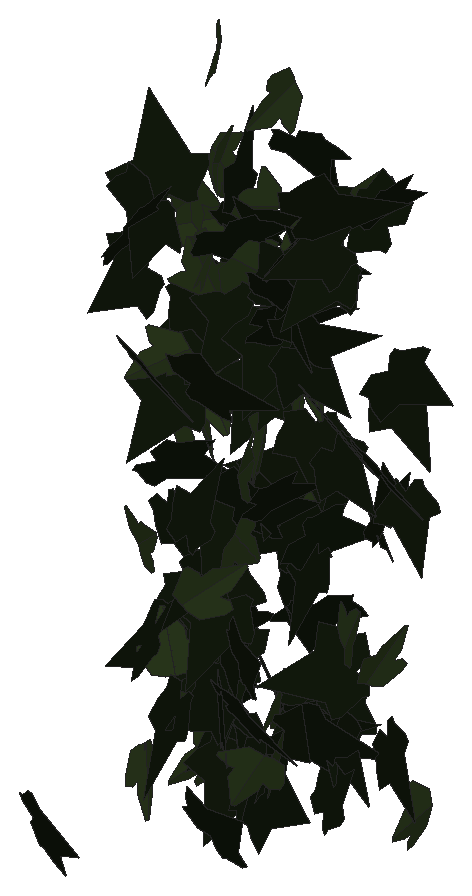
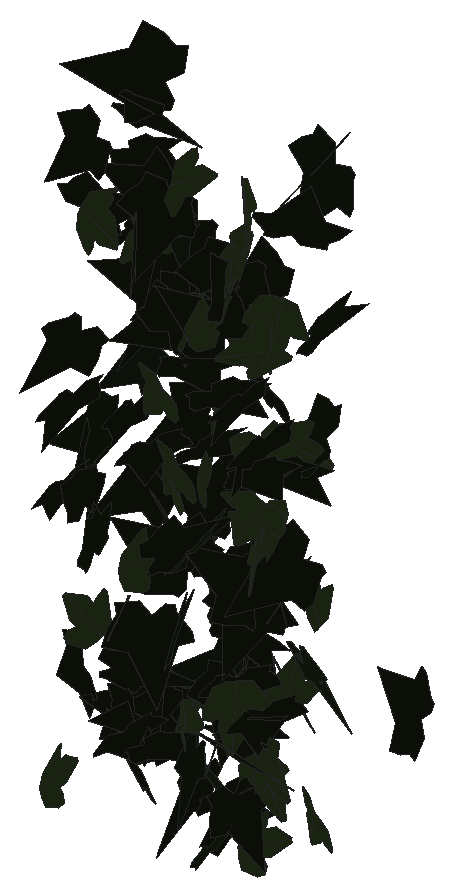
# SketchUp Ruby script. Lengths in inches.
U = 1.inch
M = Sketchup.active_model
def pt(a) = Geom::Point3d.new(a.map { |v| v * U })
def face(e, loops, mat)
  f = e.add_face(loops[0].map { |a| pt(a) })
  loops[1..].each { |l| e.add_face(l.map { |a| pt(a) }).erase! }
  f.material = f.back_material = mat if mat
  f
end
# faces: each face lists its corners as indices into pts; further lists are holes
def faces(e, pts, list, mat = nil) = list.each { |f| face(e, (f[0].is_a?(Array) ? f : [f]).map { |l| l.map { |i| pts[i] } }, mat) }
# xy, xz, yz: faces in a plane at the given z, y or x. An outline is a flat list of corners, or four numbers for a rectangle; further outlines are holes
def ring(l) = l.size == 4 ? [[l[0], l[1]], [l[2], l[1]], [l[2], l[3]], [l[0], l[3]]] : l.each_slice(2).to_a
def flat(e, list, mat, &to3) = list.each { |f| face(e, (f[0].is_a?(Array) ? f : [f]).map { |l| ring(l).map { |u, v| to3.(u, v) } }, mat) }
def xy(e, z, list, mat = nil) = flat(e, list, mat) { |x, y| [x, y, z] }
def xz(e, y, list, mat = nil) = flat(e, list, mat) { |x, z| [x, y, z] }
def yz(e, x, list, mat = nil) = flat(e, list, mat) { |y, z| [x, y, z] }
def lines(e, pts, list) = list.each { |a, b| e.add_line(pt(pts[a]), pt(pts[b])) }
# prism: a flat outline (further loops are holes) pulled along v
def prism(e, loops, v, mat = nil)
  f = face(e, loops, mat); d = Geom::Vector3d.new(v.map { |x| x * U })
  f.pushpull(f.normal.samedirection?(d) ? d.length : -d.length)
end
def box(e, o, s, mat = nil) = prism(e, [[o, [o[0] + s[0], o[1], o[2]], [o[0] + s[0], o[1] + s[1], o[2]], [o[0], o[1] + s[1], o[2]]]], [0, 0, s[2]], mat)
def at(x, y, z, deg = 0) = Geom::Transformation.translation(pt([x, y, z])) * Geom::Transformation.rotation(ORIGIN, Z_AXIS, deg.degrees)
def axes(o, x, y, z) = Geom::Transformation.new([*x, 0, *y, 0, *z, 0, *pt(o).to_a, 1])
def part(name) = M.definitions.add(name)
# library, detail: a bought-in or finely detailed component or shape, given as its bounding box
def library(name, o, s) = part(name).tap { |d| box(d.entities, o, s) }
def detail(e, o, s) = box(e.add_group.entities, o, s)
def put(e, d, t, mat = nil) = e.add_instance(d, t).tap { |i| i.material = mat if mat }
def group(e, t, mat = nil) = e.add_group.tap { |g| g.transformation = t; g.material = mat if mat }.entities
root = M.entities
M.materials.add("efeu1").color = [18, 25, 13]
M.materials.add("efeu2").color = [43, 57, 29]
c1 = part("ivyleaf_9")
p = [[1.54,2.16,1.25],[1.36,2.04,1.19],[-0.21,0.99,0.68],[-0.71,1.11,0.82],[-0.85,0.86,0.67],[-0.8,0.17,0.21],
  [-0.9,-0.01,0.1],[-0.67,-0.16,-0.02],[-0.08,-0.08,-0.05],[-0.03,-0.6,-0.4],[0.65,-0.88,-0.66],[0.83,-0.6,-0.49],
  [1.29,-0.42,-0.43],[1.8125,-0.07,-0.26],[1.21,0.44,0.15]]
faces(c1.entities,p,[[0,1,2,3,4,5,6,7,8,9,10,11,12,13,14]],"efeu1")
c2 = part("ivyleaf_10")
p = [[0,0.5,-0.03],[-0.0625,2.02,-0.43],[-0.19,2.01,-0.46],[-0.54,1.05,-0.29],[-0.52,0.625,-0.18],[-0.83,0.76,-0.28],
  [-1.16,0.64,-0.33],[-1.15,0.33,-0.24],[-0.77,-0.39,0.02],[-0.3,-0.51,0.16],[0.04,-0.48,0.23],[-0.02,2.01,-0.4375],
  [-0.06,2.01,-0.43],[0.04,-0.49,0.23],[0.67,-0.49,0.14],[1.38,0.36,-0.2],[1.375,0.51,-0.24],[0.81,0.65,-0.19],
  [0.62,0.59,-0.15],[0.6,1.09,-0.28],[0.5,1.23,-0.31]]
faces(c2.entities,p,[[0,1,2,3,4,5,6,7,8,9,10],[11,12,0,13,14,15,16,17,18,19,20]],"efeu2")
put(root,c1,axes([595.48,110.51,244.9],[0.88485,-0.15593,-1.12311],[1.13319,0.07154,0.88285],[-0.03985,-1.42802,0.16687]))
put(root,c1,axes([601.48,113.1,259.54],[-0.71196,0.76537,0.62727],[0.41363,-0.47184,1.04519],[0.89899,0.82324,0.01588]))
put(root,c1,axes([601.91,114.12,244.89],[-0.22916,-0.31013,1.32319],[0.92008,-1.023,-0.08042],[1.00024,0.86996,0.37713]))
put(root,c2,axes([601.9,113.08,256.53],[-0.35997,-0.62765,0.98561],[0.44421,0.88038,0.72287],[-1.08076,0.5709,-0.03116]))
put(root,c1,axes([597.82,115.31,272.85],[-0.11553,-1.26306,0.82528],[0.12793,-0.83291,-1.25683],[1.50334,-0.02618,0.17038]))
put(root,c1,axes([598.12,113.11,272.44],[0.25002,1.19564,0.84834],[0.18461,0.82806,-1.22147],[-1.45436,0.31065,-0.00921]))
put(root,c1,axes([600.68,114.51,265.58],[0.71694,-0.36854,1.23408],[1.15291,-0.44593,-0.80295],[0.57409,1.35577,0.07136]))
put(root,c1,axes([606.95,116.13,273.625],[-1.14976,-0.04668,0.44239],[-0.44244,-0.00738,-1.15067],[0.04622,-1.23191,-0.00987]))
put(root,c1,axes([605.85,115.38,274.94],[0.62781,0.10855,1.36523],[1.341,0.25627,-0.63705],[-0.27813,1.48065,0.01017]))
put(root,c1,axes([598.17,116.54,248.71],[-1.12531,0.13238,-0.89166],[0.86892,-0.22032,-1.12931],[-0.23994,-1.41874,0.09218]))
put(root,c1,axes([606.21,116.9,272.11],[-0.87853,-0.8025,0.25143],[-0.17708,-0.17892,-1.18982],[0.82211,-0.89611,0.0124]))
put(root,c2,axes([602.14,116.93,247.07],[-0.84663,-0.61483,0.59175],[-0.44597,-0.39188,-1.04522],[0.72752,-0.9557,0.0479]))
put(root,c1,axes([600.79,117.35,251.24],[0.05702,-0.08152,1.19859],[0.51651,-1.08171,-0.09814],[1.08465,0.51939,-0.01627]))
put(root,c1,axes([595.08,118.2,267.45],[-0.38306,-0.79546,1.00401],[-0.36805,-0.9354,-0.88152],[1.22691,-0.52896,0.04903]))
put(root,c1,axes([602.68,116.29,259.875],[0.58429,0.60526,0.85788],[0.46836,0.72841,-0.83292],[-0.93965,0.73943,0.11829]))
put(root,c1,axes([599.11,118.07,248.75],[0.08697,-0.22108,-1.27596],[1.25601,-0.29695,0.13706],[-0.31528,-1.24397,0.19405]))
put(root,c2,axes([601.49,116.76,260.67],[-0.08787,0.27007,1.15744],[-0.77353,0.86816,-0.2613],[-0.90236,-0.77051,0.11128]))
put(root,c1,axes([600.02,117.85,248.59],[0.90893,-0.64915,0.79734],[0.66494,-0.44059,-1.1167],[0.78421,1.12596,0.02272]))
put(root,c1,axes([602.58,117.15,269.81],[1.27041,0.34341,-0.24807],[-0.24015,-0.06221,-1.31601],[-0.34899,1.29291,0.00257]))
put(root,c1,axes([596.16,117.58,250.74],[-0.97894,0.88801,0.16646],[-0.12954,0.10496,-1.32166],[-0.89414,-0.98743,0.00922]))
put(root,c2,axes([600.67,117.37,257.02],[0.00862,-0.92068,-0.76166],[0.16322,0.75545,-0.91133],[1.1837,-0.09746,0.13121]))
put(root,c1,axes([602.125,118.28,268.66],[-0.02294,0.0327,-1.28813],[1.28617,0.07876,-0.02091],[0.07819,-1.28593,-0.03403]))
put(root,c1,axes([603.65,118.24,271.14],[0.49604,-0.24499,1.08564],[0.93853,-0.54673,-0.5522],[0.59815,1.06101,-0.03387]))
put(root,c1,axes([598.4,119.2,247.88],[-0.28487,-0.62266,1.06046],[-0.47461,-0.94854,-0.68444],[1.13448,-0.55318,-0.02005]))
put(root,c1,axes([596.49,117.95,271.82],[-1.36035,-0.41519,0.29721],[0.28943,0.06974,1.42219],[-0.42065,1.39069,0.01741]))
put(root,c1,axes([603.8,118.64,256.65],[-1.03975,0.04671,-0.76432],[0.75984,-0.09692,-1.03957],[-0.09497,-1.28681,0.05056]))
put(root,c2,axes([594.58,118.73,243.9],[0.92188,-0.37775,0.74099],[0.68439,-0.28405,-0.99627],[0.47262,1.14815,-0.00269]))
put(root,c2,axes([594.45,118.72,254.04],[-0.72953,0.19166,0.88927],[0.85302,-0.25191,0.75409],[0.31605,1.1223,0.0174]))
put(root,c1,axes([594.22,118.63,262.75],[0.95495,-0.66061,0.53058],[0.43961,-0.29713,-1.16117],[0.72434,1.05126,0.00523]))
put(root,c1,axes([603.1,118.17,266.82],[0.48098,-0.06964,1.19668],[1.19796,-0.01764,-0.48252],[0.04236,1.2896,0.05802]))
put(root,c1,axes([604.23,119.62,270.13],[-0.45047,-0.94656,0.77094],[-0.21018,-0.74934,-1.04286],[1.20256,-0.48554,0.10651]))
put(root,c2,axes([596.29,118.5,249.23],[0.6545,0.96806,0.06775],[-0.0525,-0.04628,1.16842],[0.96901,-0.65636,0.01754]))
put(root,c1,axes([603.14,118.33,266.3],[0.42444,-0.76433,-1.01895],[-0.33985,0.96715,-0.86703],[1.22759,0.53202,0.11227]))
put(root,c1,axes([603.45,118.7,264.02],[1.24959,-0.56664,0.11152],[0.10363,-0.0415,-1.37205],[0.56814,1.25386,0.00499]))
put(root,c1,axes([597.48,119.6,253.69],[-0.02379,0.07537,-1.1814],[0.47562,-1.08146,-0.07857],[-1.08405,-0.47614,-0.00854]))
put(root,c1,axes([599.53,118.83,257.48],[0.36313,-0.28023,1.35676],[1.31806,-0.36211,-0.42756],[0.42669,1.35704,0.16608]))
put(root,c1,axes([602.85,118.39,271.36],[-0.34607,1.1536,0.10618],[-0.04311,0.09791,-1.20432],[-1.15767,-0.3485,0.01311]))
put(root,c1,axes([598.33,119.5,252.24],[-1.16934,-0.58558,-0.35614],[0.3581,0.0785,-1.30488],[0.58438,-1.21985,0.08699]))
put(root,c1,axes([595.65,119.89,261.3],[-1.06583,-0.73271,0.05135],[-0.0269,-0.0515,-1.29311],[0.73401,-1.06583,0.02718]))
put(root,c1,axes([598.48,120.14,244.42],[-0.54184,-1.17495,0.20217],[-0.05531,-0.19706,-1.29348],[1.19094,-0.54372,0.03191]))
put(root,c2,axes([595.33,120.03,262.75],[-0.44485,-0.28803,1.0474],[-0.65665,-0.83032,-0.50722],[0.86534,-0.77814,0.15355]))
put(root,c1,axes([600.03,119.47,244.68],[-1.15305,0.7623,0.16219],[-0.13378,0.09174,-1.38225],[-0.7678,-1.16078,-0.00273]))
put(root,c1,axes([603.49,118.55,257.63],[-0.08354,0.41063,-1.21943],[-0.17231,1.20742,0.4184],[1.27512,0.19007,-0.02335]))
put(root,c1,axes([595.1875,119.71,255.55],[0.77947,-0.96786,-0.28075],[-0.17077,0.22294,-1.24269],[0.99318,0.79793,0.00667]))
put(root,c1,axes([598.14,120.4375,256.3],[-0.82316,-1.11408,-0.13571],[0.09135,0.10123,-1.38513],[1.11859,-0.82811,0.01326]))
put(root,c1,axes([600.4,120.375,265.22],[-0.86617,-0.93476,-0.12222],[0.07691,0.09536,-1.27435],[0.93957,-0.86954,-0.00837]))
put(root,c2,axes([600.69,120.29,246.25],[0.63115,-0.95708,0.418],[0.2287,-0.34989,-1.14645],[1.01903,0.67131,-0.0016]))
put(root,c1,axes([604.07,119.58,261.23],[0.37146,-0.75058,-0.78672],[-0.27821,0.73808,-0.83553],[1.05114,0.4606,0.05687]))
put(root,c2,axes([599.27,120.67,260.02],[0.12504,-0.45101,1.17667],[0.81726,-0.87103,-0.4207],[0.95919,0.80093,0.20506]))
put(root,c2,axes([596.97,119.86,268.23],[0.76699,-0.80704,-0.3962],[-0.27793,0.28244,-1.11335],[0.85501,0.81577,-0.00649]))
put(root,c2,axes([596.96,120.17,266.67],[-1.02966,-0.39652,-0.41797],[-0.39178,-0.1457,1.10336],[-0.42241,1.10167,-0.00452]))
put(root,c1,axes([600.9375,118.93,266.5],[0.81658,0.46889,1.0733],[0.79029,0.7451,-0.92677],[-0.86446,1.1241,0.1666]))
put(root,c1,axes([606.17,120.42,248.03],[-0.14185,-0.21312,-1.29929],[1.31012,0.10716,-0.16061],[0.13098,-1.30261,0.19936]))
put(root,c1,axes([598.55,119.25,269.9],[0.81941,1.17922,-0.02418],[-0.01251,-0.02075,-1.43596],[-1.1794,0.8195,-0.00157]))
put(root,c1,axes([600.5,119.19,244.23],[0.36663,-0.23977,-1.36091],[-0.86458,1.05857,-0.41942],[1.078,0.93055,0.12646]))
put(root,c2,axes([602.3,119.66,270.9375],[0.49998,0.59753,0.91656],[0.401,0.83753,-0.76475],[-1.018,0.62338,0.14891]))
put(root,c1,axes([606.29,119.42,273.72],[0.41575,0.77698,0.75727],[0.3268,0.68362,-0.88084],[-1.03458,0.52818,0.02608]))
put(root,c1,axes([601.64,120.28,247.21],[0.62444,0.40686,-1.26793],[1.06148,0.69347,0.74529],[0.80401,-1.23153,0.00079]))
put(root,c1,axes([602.75,120.56,243.61],[-0.45394,0.82052,0.827],[0.41111,-0.71764,0.93767],[1.09003,0.61236,-0.00924]))
put(root,c2,axes([598.72,120.12,268.26],[-0.5851,-0.5992,-0.91061],[0.60193,0.68404,-0.83688],[0.90881,-0.83884,-0.03197]))
put(root,c1,axes([596.89,121.18,248.15],[-0.66334,-0.76295,-0.71327],[0.7905,0.18549,-0.93357],[0.6826,-0.95622,0.388]))
put(root,c1,axes([601.35,119.81,247.15],[0.26985,0.68474,-1.10394],[0.32651,1.05556,0.73454],[1.25736,-0.42106,0.04618]))
put(root,c1,axes([598.84,121.53,261.98],[-0.53465,-1.05883,0.3155],[-0.00028,-0.35036,-1.17632],[1.10483,-0.51247,0.15237]))
put(root,c1,axes([597.91,121.6,265.0625],[-0.96319,-0.94532,0.21405],[-0.08791,-0.21532,-1.34651],[0.96526,-0.9629,0.09096]))
put(root,c1,axes([597.79,120.2,249.91],[0.71912,-0.28563,-1.09556],[-0.94359,0.56605,-0.76695],[0.62568,1.18194,0.10255]))
put(root,c1,axes([604.57,120.88,260.64],[0.99083,-0.55712,0.409],[0.3551,-0.20295,-1.13671],[0.59293,1.05254,-0.0027]))
put(root,c2,axes([595.79,121.72,243.3125],[0.01014,-0.20831,1.1603],[0.07999,-1.15755,-0.20851],[1.17614,0.08052,0.00418]))
put(root,c1,axes([601.65,121.27,260.97],[-0.20012,-1.12042,-0.36539],[0.06658,0.35928,-1.13815],[1.17661,-0.21089,0.00225]))
put(root,c1,axes([596.5625,120.47,255.12],[0.60232,1.10718,-0.39853],[0.20457,0.34236,1.26031],[1.1588,-0.63593,-0.01534]))
put(root,c2,axes([601.18,121.23,263.75],[0.87424,-0.10146,0.7759],[0.76911,-0.10293,-0.88005],[0.14417,1.16435,-0.01019]))
put(root,c2,axes([600.07,120.8125,247.95],[0.37822,-1.08268,-0.50877],[-0.12689,0.49427,-1.14616],[1.18952,0.39698,0.0395]))
put(root,c1,axes([600.52,121.28,267.09],[0.2281,-0.02764,1.34009],[-1.31722,0.24697,0.2293],[-0.24808,-1.33674,0.01465]))
put(root,c2,axes([595.85,121.0625,246.94],[-0.95745,-0.05087,0.76789],[-0.75285,-0.1922,-0.95143],[0.15954,-1.21219,0.11863]))
put(root,c1,axes([602.66,121.26,247.3],[-0.29039,-0.12194,-1.27016],[1.22358,0.34291,-0.31266],[0.36196,-1.257,0.03792]))
put(root,c1,axes([594.36,120.13,257.3],[0.98695,0.78539,0.59876],[0.46292,0.37986,-1.26128],[-0.87239,1.09009,0.00811]))
put(root,c1,axes([598.87,122.11,257.01],[-0.0921,-1.05107,0.83425],[0.25227,-0.83486,-1.02399],[1.31798,0.08635,0.2543]))
put(root,c1,axes([596.42,120.59,254.98],[1.0439,0.72586,-0.30831],[-0.26418,-0.16006,-1.27132],[-0.74306,1.07665,0.01886]))
put(root,c1,axes([603.13,121.8,249.64],[-1.03128,-0.12095,0.87929],[-0.86217,-0.18364,-1.03647],[0.21081,-1.34275,0.06254]))
put(root,c1,axes([600.31,120.64,255.04],[-0.16235,-0.17523,1.44747],[1.39415,0.40773,0.20573],[-0.42686,1.39831,0.1214]))
put(root,c2,axes([605.09,120.96,250.63],[-0.01239,-1.00098,0.5724],[0.0537,0.57131,1.00024],[-1.15183,0.0374,0.04048]))
put(root,c2,axes([595.6,121.02,247.5],[-0.48428,0.05314,1.09712],[-1.08355,0.17343,-0.48669],[-0.18005,-1.18664,-0.022]))
put(root,c1,axes([597.4,120.67,250.36],[0.45367,1.17888,-0.0892],[-0.04321,-0.07895,-1.2631],[-1.18146,0.45556,0.01195]))
put(root,c2,axes([596.98,120.76,272.31],[-0.22217,0.99219,0.58733],[-0.22488,0.54936,-1.01311],[-1.13085,-0.30417,0.08608]))
put(root,c2,axes([594.73,121.19,269.93],[-1.23067,-0.17092,-0.1005],[0.10018,0.0093,-1.24247],[0.17111,-1.23473,0.00456]))
put(root,c2,axes([597.12,120.58,272.08],[-0.14402,0.49585,1.05803],[-0.64285,0.85657,-0.48894],[-0.97572,-0.63754,0.16596]))
put(root,c1,axes([605.1,121.49,271.625],[-0.37691,0.14768,1.21148],[-1.18445,0.26138,-0.40037],[-0.2942,-1.24154,0.05982]))
put(root,c1,axes([596.03,122.29,249.35],[-0.80947,-0.86204,0.34152],[-0.0801,-0.38664,-1.1658],[0.92376,-0.78891,0.19818]))
put(root,c1,axes([596.37,121.9,251.52],[-0.33636,-1.09173,-0.47699],[0.12937,0.45923,-1.14232],[1.18434,-0.36022,-0.01069]))
put(root,c1,axes([604.85,121.875,257.32],[0.12726,0.84899,0.91133],[-0.44668,-0.82403,0.83003],[1.16266,-0.40951,0.21914]))
put(root,c2,axes([599.18,122.47,275.41],[0.13711,0.41133,-1.16672],[-0.33177,-1.11863,-0.43336],[-1.19178,0.35873,-0.01359]))
put(root,c1,axes([596.55,122.65,244.84],[0.16197,-0.2751,-1.16488],[0.45467,-1.07324,0.31668],[-1.1072,-0.48096,-0.04037]))
put(root,c2,axes([594.98,120.81,259.18],[-0.14476,0.24372,1.22244],[-0.5656,1.08383,-0.28306],[-1.11079,-0.58363,-0.01518]))
put(root,c1,axes([594.78,122.07,250.5],[-0.22371,-1.16651,-0.38425],[0.04377,0.38275,-1.18744],[1.22738,-0.22626,-0.02768]))
put(root,c1,axes([601.58,121.36,252.41],[0.4616,1.13972,-0.5279],[-0.29603,-0.44786,-1.22577],[-1.22066,0.53961,0.09764]))
put(root,c2,axes([603.48,120.94,251.66],[0.11279,0.0952,-1.13734],[-0.20785,1.12548,0.07359],[1.12223,0.19889,0.12794]))
put(root,c1,axes([605.74,121.16,264.99],[0.04898,-0.17499,-1.20851],[-0.17409,1.19612,-0.18025],[1.20863,0.17938,0.02301]))
put(root,c1,axes([600.69,122.71,247.07],[-0.79162,-0.77595,0.34486],[-0.21043,-0.2775,-1.10743],[0.82264,-0.81767,0.04858]))
put(root,c1,axes([600.0625,121.82,251.92],[0.09729,-0.91045,0.92088],[-0.05059,0.9201,0.91503],[-1.29398,-0.10443,0.03347]))
put(root,c1,axes([597.26,122.04,247.91],[-0.98465,0.63925,0.6458],[-0.72633,0.01851,-1.12576],[-0.54602,-1.17739,0.33293]))
put(root,c1,axes([594.94,122.7,262.67],[-0.66246,-0.97908,-0.01181],[0.00807,0.0088,-1.18213],[0.97911,-0.66251,0.00175]))
put(root,c2,axes([605.9,122.96,243.48],[-0.03313,0.02076,1.20918],[0.4688,-1.11483,0.03198],[1.1148,0.46943,0.02248]))
put(root,c2,axes([599.53,122.14,259.59],[0.85253,-0.79065,0.01438],[-0.00909,0.01134,1.16272],[-0.79073,-0.85257,0.00213]))
put(root,c2,axes([603.77,122.85,272.28],[0.10314,-0.98126,0.73885],[0.10301,-0.73193,-0.98644],[1.22399,0.14428,0.02076]))
put(root,c1,axes([601.92,122.77,247.29],[-0.24781,-1.17538,-0.04486],[0.00902,0.04394,-1.20122],[1.1762,-0.24797,-0.00024]))
put(root,c1,axes([597.06,122.16,268.4],[0.22754,-0.37692,1.15478],[1.19574,-0.1375,-0.28049],[0.21403,1.16893,0.33937]))
put(root,c2,axes([596.29,122.23,250.81],[-0.74945,-1.01351,-0.09522],[0.05651,0.07664,-1.26051],[1.0164,-0.75158,-0.00013]))
put(root,c2,axes([594.96,121.47,268.12],[0.00317,-0.0802,1.18514],[0.38678,1.12063,0.0748],[-1.12312,0.38569,0.02911]))
put(root,c2,axes([594.93,122.17,260.52],[0.98299,0.42679,0.65811],[0.60637,0.25584,-1.07162],[-0.49756,1.15495,-0.00581]))
put(root,c1,axes([605.39,122.61,258.46],[0.15948,-1.14754,-0.25465],[-0.05063,0.25004,-1.15847],[1.17436,0.16662,-0.01536]))
put(root,c1,axes([596.14,122.32,245.91],[-0.26736,1.00407,-0.63107],[0.19788,-0.60007,-1.03858],[-1.16929,-0.33114,-0.03146]))
put(root,c1,axes([597.15,121.8,270.09],[-0.00817,-0.61423,1.11132],[0.40605,1.05172,0.58427],[-1.20309,0.35914,0.18965]))
put(root,c2,axes([595.36,121.77,258.7],[-0.64025,0.67585,0.72772],[-0.51993,0.50961,-0.93072],[-0.84618,-0.8245,0.02126]))
put(root,c1,axes([600.28,121.82,273.8],[1.06916,0.62461,-0.33341],[-0.29321,-0.15903,-1.2382],[-0.64446,1.10859,0.01023]))
put(root,c1,axes([595.72,122.4375,265.93],[0.32854,-0.9976,-0.52329],[-0.10687,0.51503,-1.04895],[1.12144,0.34135,0.05334]))
put(root,c1,axes([599.56,123.34,257.13],[-0.38882,-0.15956,1.27167],[-1.00017,-0.7932,-0.40533],[0.80142,-1.06732,0.11112]))
put(root,c1,axes([603.21,123.29,256.14],[0.05006,-0.49492,1.10131],[0.36906,-1.04323,-0.4856],[1.14962,0.35646,0.10793]))
put(root,c2,axes([597.4,123.32,269.01],[-0.03121,0.45651,1.088],[0.12044,-1.08147,0.45722],[1.17373,0.12311,-0.01798]))
put(root,c1,axes([594.35,122.625,264.32],[0.33015,-1.10305,-0.62909],[-0.15795,0.60928,-1.15121],[1.25997,0.36541,0.02053]))
put(root,c1,axes([596.54,123.58,243.77],[-0.11467,-0.79523,0.86357],[0.23124,-0.86598,-0.76674],[1.15094,0.09475,0.24009]))
put(root,c1,axes([598.3,122.43,247.45],[0.80871,-0.07015,-0.84859],[-0.8383,0.13956,-0.81044],[0.14926,1.16389,0.04603]))
put(root,c2,axes([600.71,123.79,256.4],[-0.03583,-0.00062,1.24994],[0.17243,-1.2385,0.00433],[1.23799,0.17248,0.03557]))
put(root,c2,axes([595.41,122.5625,276.25],[0.46201,-0.90969,-0.6142],[-0.20331,0.58394,-1.0178],[1.07863,0.49971,0.07124]))
put(root,c2,axes([598.68,123.16,261.5625],[0.92648,-0.17198,0.81089],[0.79188,-0.1759,-0.94206],[0.24506,1.21859,-0.02154]))
put(root,c1,axes([604.69,122.92,263.09],[0.26781,-1.07085,-0.629],[-0.14591,0.61187,-1.10381],[1.23331,0.30492,0.006]))
put(root,c1,axes([601.73,122.26,271.81],[0.05067,0.17666,-1.12335],[-1.0576,0.42052,0.01843],[0.41786,1.0429,0.18286]))
